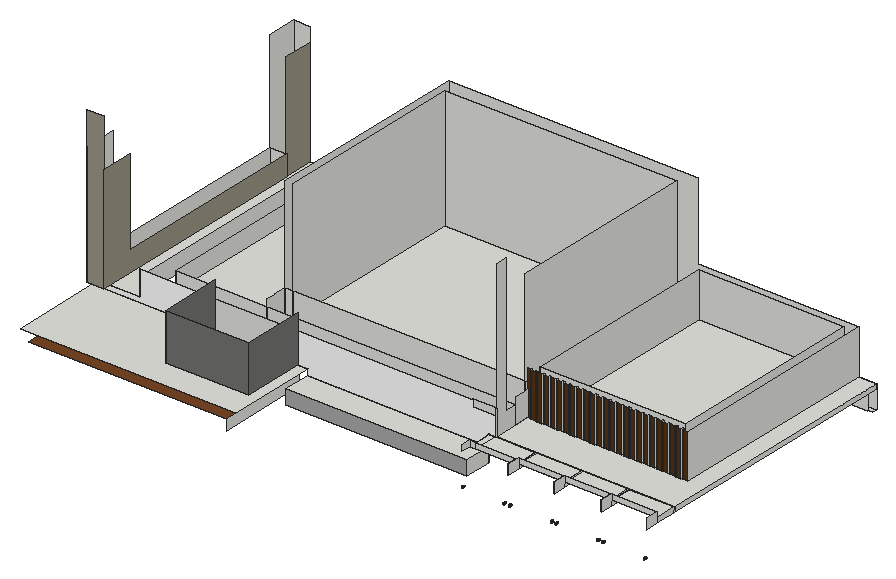
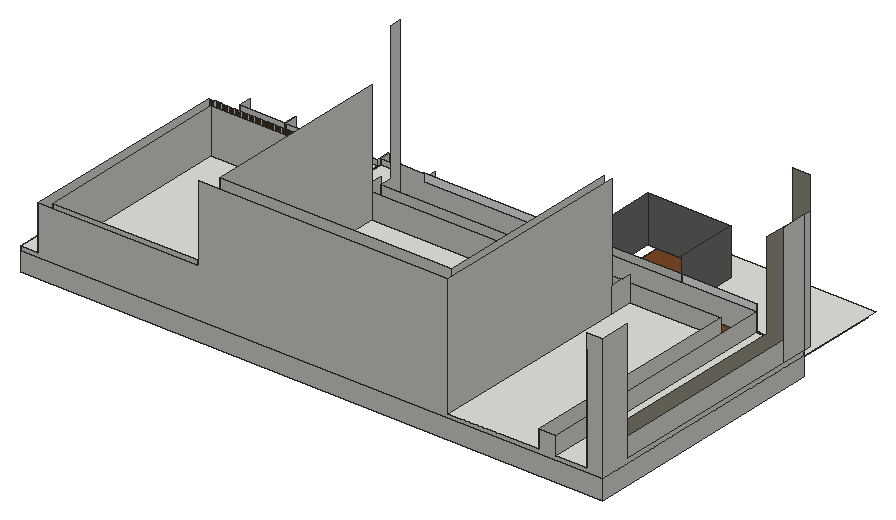
# SketchUp Ruby script. Lengths in inches.
U = 1.inch
M = Sketchup.active_model
def pt(a) = Geom::Point3d.new(a.map { |v| v * U })
def face(e, loops, mat)
  f = e.add_face(loops[0].map { |a| pt(a) })
  loops[1..].each { |l| e.add_face(l.map { |a| pt(a) }).erase! }
  f.material = f.back_material = mat if mat
  f
end
# faces: each face lists its corners as indices into pts; further lists are holes
def faces(e, pts, list, mat = nil) = list.each { |f| face(e, (f[0].is_a?(Array) ? f : [f]).map { |l| l.map { |i| pts[i] } }, mat) }
# xy, xz, yz: faces in a plane at the given z, y or x. An outline is a flat list of corners, or four numbers for a rectangle; further outlines are holes
def ring(l) = l.size == 4 ? [[l[0], l[1]], [l[2], l[1]], [l[2], l[3]], [l[0], l[3]]] : l.each_slice(2).to_a
def flat(e, list, mat, &to3) = list.each { |f| face(e, (f[0].is_a?(Array) ? f : [f]).map { |l| ring(l).map { |u, v| to3.(u, v) } }, mat) }
def xy(e, z, list, mat = nil) = flat(e, list, mat) { |x, y| [x, y, z] }
def xz(e, y, list, mat = nil) = flat(e, list, mat) { |x, z| [x, y, z] }
def yz(e, x, list, mat = nil) = flat(e, list, mat) { |y, z| [x, y, z] }
def lines(e, pts, list) = list.each { |a, b| e.add_line(pt(pts[a]), pt(pts[b])) }
# prism: a flat outline (further loops are holes) pulled along v
def prism(e, loops, v, mat = nil)
  f = face(e, loops, mat); d = Geom::Vector3d.new(v.map { |x| x * U })
  f.pushpull(f.normal.samedirection?(d) ? d.length : -d.length)
end
def box(e, o, s, mat = nil) = prism(e, [[o, [o[0] + s[0], o[1], o[2]], [o[0] + s[0], o[1] + s[1], o[2]], [o[0], o[1] + s[1], o[2]]]], [0, 0, s[2]], mat)
def at(x, y, z, deg = 0) = Geom::Transformation.translation(pt([x, y, z])) * Geom::Transformation.rotation(ORIGIN, Z_AXIS, deg.degrees)
def axes(o, x, y, z) = Geom::Transformation.new([*x, 0, *y, 0, *z, 0, *pt(o).to_a, 1])
def part(name) = M.definitions.add(name)
# library, detail: a bought-in or finely detailed component or shape, given as its bounding box
def library(name, o, s) = part(name).tap { |d| box(d.entities, o, s) }
def detail(e, o, s) = box(e.add_group.entities, o, s)
def put(e, d, t, mat = nil) = e.add_instance(d, t).tap { |i| i.material = mat if mat }
def group(e, t, mat = nil) = e.add_group.tap { |g| g.transformation = t; g.material = mat if mat }.entities
root = M.entities
M.materials.add("[0030_OldLace]").color = [86, 53, 24]
M.materials.add("[0128_White]").color = [255, 255, 255]
M.materials.add("[Color M03]").color = [170, 170, 170]
M.materials.add("[Concrete Tile]").color = [155, 150, 134]
M.materials.add("[Metal Seamed]").color = [116, 117, 113]
M.materials.add("[Wood Veneer 01]").color = [120, 70, 37]
xy(root,95.79,[[684.16,846.1,784.44,851.0625]])
xy(root,99.26,[[621.47,810.97,848.72,845.35]],"[Wood Veneer 01]")
xy(root,101.375,[[545.16,845.35,610.53,846.1],[352.17,846.1,352.17,1160.85,1080.92,1160.85,1080.92,1155.13,357.89,1155.13,357.89,851.0625,545.16,851.0625,545.16,846.1],[545.16,846.1,610.53,851.0625]])
xy(root,101.78,[[374.83,845.35,499.71,851.0625]])
xy(root,114.25,[[363.11,732.28,610.53,845.35]],"[Wood Veneer 01]")
xy(root,117.26,[[621.47,810.97,848.72,845.35]])
xy(root,125.1875,[[352.17,732.28,621.47,732.28,621.47,845.35,609.54,845.35,609.54,767.72,505.35,767.72,505.35,845.35,352.17,845.35],[352.17,845.35,621.47,846.1]])
xy(root,131.1875,[[848.72,814.22,849.1875,844.47],[849.1875,814.22,857.125,844.47],[857.125,814.22,906.77,844.47],[907.71,817.6,964.82,844.47],[965.89,817.6,1022.875,844.47],
  [1024.1875,817.6,1080.92,844.47],[352.17,837.03,372.92,845.35],[848.72,844.47,849.1875,845.35],[849.1875,844.47,857.125,845.35],[857.125,844.47,1080.92,846.1],
  [352.17,845.35,372.92,846.1],[372.92,845.35,411.09,846.1],[848.72,845.35,849.1875,846.1],[849.1875,845.35,857.125,846.1],[352.17,846.1,372.92,877.14],
  [372.92,846.1,411.09,846.1,411.09,1160.85,372.3,1160.85,372.3,1122.97,372.92,1122.97],[857.125,846.1,1080.92,846.1,1080.92,1160.85,1058.5,1160.85,1058.5,893.65,1052.35,893.65,1052.35,895.71,1050.1875,895.71,1050.1875,893.65,1044.04,893.65,1044.04,895.71,1041.875,895.71,1041.875,894.34,1035.73,894.34,1035.73,895.71,1033.5625,895.71,1033.5625,894.34,1027.41,894.34,1027.41,895.71,1025.25,895.71,1025.25,894.34,1019.1,894.34,1019.1,895.71,1016.9375,895.71,1016.9375,894.34,1010.79,894.34,1010.79,895.71,1008.625,895.71,1008.625,894.34,1002.48,894.34,1002.48,895.71,1000.3125,895.71,1000.3125,894.34,994.16,894.34,994.16,895.71,992,895.71,992,894.34,985.85,894.34,985.85,895.71,983.6875,895.71,983.6875,894.34,977.54,894.34,977.54,895.71,975.375,895.71,975.375,894.34,969.23,894.34,969.23,895.71,967.0625,895.71,967.0625,894.34,960.91,894.34,960.91,895.71,958.75,895.71,958.75,894.34,952.6,894.34,952.6,895.71,950.4375,895.71,950.4375,894.34,944.29,894.34,944.29,895.71,942.125,895.71,942.125,894.34,935.98,894.34,935.98,895.71,933.8125,895.71,933.8125,894.34,927.66,894.34,927.66,895.71,925.5,895.71,925.5,894.34,919.35,894.34,919.35,895.71,917.1875,895.71,917.1875,894.34,911.04,894.34,911.04,895.71,908.875,895.71,908.875,894.34,902.73,894.34,902.73,895.71,900.5625,895.71,900.5625,894.34,894.41,894.34,894.41,895.71,892.25,895.71,892.25,894.34,886.1,894.34,886.1,895.71,883.9375,895.71,883.9375,894.34,877.79,894.34,877.79,895.71,875.625,895.71,875.625,894.34,869.48,894.34,869.48,895.71,867.3125,895.71,867.3125,894.34,861.16,894.34,861.16,895.71,857.125,895.71],[352.17,877.14,372.92,1122.97],[431.5,877.14,545.16,1160.85],[545.16,877.14,857.125,905.7],
  [865.59,904.18,1047.28,1152.375],[554.54,905.7,844.86,1143.26]])
xz(root,767.72,[[505.35,125.1875,609.54,183.3125]],"[Metal Seamed]")
xz(root,799.91,[[851.55,91.63,851.84,91.67,852.11,91.78,852.34,91.96,852.52,92.19,852.63,92.46,852.67,92.75,852.63,93.04,852.52,93.32,852.34,93.55,852.11,93.73,851.84,93.84,851.55,93.88,851.25,93.84,850.98,93.73,850.75,93.55,850.57,93.32,850.46,93.04,850.42,92.75,850.46,92.46,850.57,92.19,850.75,91.96,850.98,91.78,851.25,91.67],[903.73,91.63,904.02,91.67,904.3,91.78,904.53,91.96,904.71,92.19,904.82,92.46,904.86,92.75,904.82,93.04,904.71,93.32,904.53,93.55,904.3,93.73,904.02,93.84,903.73,93.88,903.44,93.84,903.17,93.73,902.9375,93.55,902.76,93.32,902.65,93.04,902.61,92.75,902.65,92.46,902.76,92.19,902.9375,91.96,903.17,91.78,903.44,91.67],[910.53,91.63,910.82,91.67,911.1,91.78,911.33,91.96,911.51,92.19,911.62,92.46,911.66,92.75,911.62,93.04,911.51,93.32,911.33,93.55,911.1,93.73,910.82,93.84,910.53,93.88,910.24,93.84,909.97,93.73,909.74,93.55,909.56,93.32,909.45,93.04,909.41,92.75,909.45,92.46,909.56,92.19,909.74,91.96,909.97,91.78,910.24,91.67],[962.72,91.63,963.01,91.67,963.28,91.78,963.52,91.96,963.7,92.19,963.81,92.46,963.85,92.75,963.81,93.04,963.7,93.32,963.52,93.55,963.28,93.73,963.01,93.84,962.72,93.88,962.43,93.84,962.16,93.73,961.93,93.55,961.75,93.32,961.63,93.04,961.6,92.75,961.63,92.46,961.75,92.19,961.93,91.96,962.16,91.78,962.43,91.67],[968.71,91.63,969,91.67,969.27,91.78,969.5,91.96,969.68,92.19,969.8,92.46,969.83,92.75,969.8,93.04,969.68,93.32,969.5,93.55,969.27,93.73,969,93.84,968.71,93.88,968.42,93.84,968.15,93.73,967.91,93.55,967.74,93.32,967.62,93.04,967.58,92.75,967.62,92.46,967.74,92.19,967.91,91.96,968.15,91.78,968.42,91.67],
  [1020.9,91.63,1021.1875,91.67,1021.46,91.78,1021.69,91.96,1021.87,92.19,1021.98,92.46,1022.02,92.75,1021.98,93.04,1021.87,93.32,1021.69,93.55,1021.46,93.73,1021.1875,93.84,1020.9,93.88,1020.61,93.84,1020.33,93.73,1020.1,93.55,1019.92,93.32,1019.81,93.04,1019.77,92.75,1019.81,92.46,1019.92,92.19,1020.1,91.96,1020.33,91.78,1020.61,91.67],[1027.01,91.63,1027.3,91.67,1027.57,91.78,1027.81,91.96,1027.98,92.19,1028.1,92.46,1028.14,92.75,1028.1,93.04,1027.98,93.32,1027.81,93.55,1027.57,93.73,1027.3,93.84,1027.01,93.88,1026.72,93.84,1026.45,93.73,1026.21,93.55,1026.04,93.32,1025.92,93.04,1025.89,92.75,1025.92,92.46,1026.04,92.19,1026.21,91.96,1026.45,91.78,1026.72,91.67],[1079.2,91.63,1079.49,91.67,1079.76,91.78,1079.99,91.96,1080.17,92.19,1080.28,92.46,1080.32,92.75,1080.28,93.04,1080.17,93.32,1079.99,93.55,1079.76,93.73,1079.49,93.84,1079.2,93.88,1078.91,93.84,1078.64,93.73,1078.4,93.55,1078.22,93.32,1078.11,93.04,1078.07,92.75,1078.11,92.46,1078.22,92.19,1078.4,91.96,1078.64,91.78,1078.91,91.67]])
xz(root,810.97,[[621.47,99.26,848.72,117.26]],"[Color M03]")
xz(root,814.22,[[848.72,131.1875,857.125,138.0625],[857.125,131.1875,906.77,138.0625]])
xz(root,817.6,[[907.71,131.1875,964.82,138.0625],[965.89,131.1875,1022.875,138.0625],[1024.1875,131.1875,1080.92,138.0625]])
xz(root,837.03,[[352.17,131.1875,372.92,324.5625]],"[Concrete Tile]")
xz(root,845.35,[[621.47,99.26,848.72,117.26],[505.35,125.1875,609.54,162.75]])
xz(root,845.35,[[621.47,117.26,848.72,117.26,848.72,131.1875,857.125,131.1875,857.125,154.75,827.91,154.75,827.91,162.75,609.54,162.75,609.54,125.1875,621.47,125.1875],[352.17,125.1875,505.35,125.1875,505.35,162.75,411.09,162.75,411.09,131.1875,352.17,131.1875]],"[0128_White]")
xz(root,846.1,[[352.17,125.1875,352.17,131.1875,411.09,131.1875,411.09,153.5625,827.91,153.5625,827.91,163,857.125,163,857.125,131.1875,848.72,131.1875,848.72,125.1875]])
xz(root,851.0625,[[374.83,101.375,499.71,101.78]])
xz(root,877.14,[[431.5,131.1875,545.16,153.5625],[545.16,131.1875,857.125,153.5625]])
xz(root,893.65,[[1044.04,131.1875,1050.1875,186.75],[1052.35,131.1875,1058.5,186.75]],"[0030_OldLace]")
xz(root,894.34,[[861.16,131.1875,867.3125,186.75],[869.48,131.1875,875.625,186.75],[877.79,131.1875,883.9375,186.75],[886.1,131.1875,892.25,186.75],[894.41,131.1875,900.5625,186.75],
  [902.73,131.1875,908.875,186.75],[911.04,131.1875,917.1875,186.75],[919.35,131.1875,925.5,186.75],[927.66,131.1875,933.8125,186.75],[935.98,131.1875,942.125,186.75],
  [944.29,131.1875,950.4375,186.75],[952.6,131.1875,958.75,186.75],[960.91,131.1875,967.0625,186.75],[969.23,131.1875,975.375,186.75],[977.54,131.1875,983.6875,186.75],
  [985.85,131.1875,992,186.75],[994.16,131.1875,1000.3125,186.75],[1002.48,131.1875,1008.625,186.75],[1010.79,131.1875,1016.9375,186.75],[1019.1,131.1875,1025.25,186.75],
  [1027.41,131.1875,1033.5625,186.75],[1035.73,131.1875,1041.875,186.75]],"[0030_OldLace]")
xz(root,895.71,[[857.125,131.1875,861.16,186.75],[867.3125,131.1875,869.48,186.75],[875.625,131.1875,877.79,186.75],[883.9375,131.1875,886.1,186.75],[892.25,131.1875,894.41,186.75],
  [900.5625,131.1875,902.73,186.75],[908.875,131.1875,911.04,186.75],[917.1875,131.1875,919.35,186.75],[925.5,131.1875,927.66,186.75],[933.8125,131.1875,935.98,186.75],
  [942.125,131.1875,944.29,186.75],[950.4375,131.1875,952.6,186.75],[958.75,131.1875,960.91,186.75],[967.0625,131.1875,969.23,186.75],[975.375,131.1875,977.54,186.75],
  [983.6875,131.1875,985.85,186.75],[992,131.1875,994.16,186.75],[1000.3125,131.1875,1002.48,186.75],[1008.625,131.1875,1010.79,186.75],[1016.9375,131.1875,1019.1,186.75],
  [1025.25,131.1875,1027.41,186.75],[1033.5625,131.1875,1035.73,186.75],[1041.875,131.1875,1044.04,186.75],[1050.1875,131.1875,1052.35,186.75]],"[0030_OldLace]")
xz(root,904.18,[[865.59,131.1875,1047.28,186.75]])
xz(root,905.7,[[545.16,131.1875,554.54,162.75],[554.54,131.1875,844.86,162.75],[844.86,131.1875,857.125,162.75]])
xz(root,1122.97,[[352.17,131.1875,372.3,156.5],[372.3,131.1875,372.92,156.5]])
xz(root,1143.26,[[554.54,131.1875,844.86,282.75]])
xz(root,1152.375,[[865.59,131.1875,1047.28,186.75]])
xz(root,1155.13,[[357.89,101.375,1075.21,125.1875]])
xz(root,1160.85,[[352.17,101.375,1080.92,125.1875],[352.17,125.1875,352.17,282.75,372.3,282.75,372.3,131.1875,411.09,131.1875,411.09,153.5625,431.5,153.5625,431.5,131.1875,545.16,131.1875,545.16,282.75,857.125,282.75,857.125,186.75,1058.5,186.75,1058.5,131.1875,1080.92,131.1875,1080.92,125.1875]])
yz(root,352.17,[[846.1,101.375,1160.85,125.1875],[845.35,125.1875,846.1,131.1875],[846.1,125.1875,846.1,131.1875,1122.97,131.1875,1122.97,282.75,1160.85,282.75,1160.85,125.1875],[837.03,131.1875,845.35,282.75],[845.35,131.1875,877.14,282.75],
  [877.14,131.1875,1122.97,156.5]])
yz(root,357.89,[[851.0625,101.375,1155.13,125.1875]])
yz(root,372.3,[[1122.97,131.1875,1160.85,264.75]],"[Concrete Tile]")
yz(root,372.92,[[837.03,131.1875,1122.97,131.1875,1122.97,156.5,877.14,156.5,877.14,264.75,837.03,264.75]],"[Concrete Tile]")
yz(root,411.09,[[845.35,131.1875,846.1,162.75],[846.1,131.1875,1160.85,153.5625]])
yz(root,431.5,[[877.14,131.1875,1160.85,153.5625]])
yz(root,505.35,[[767.72,125.1875,845.35,183.3125]],"[Metal Seamed]")
yz(root,545.16,[[877.14,131.1875,877.14,162.125,888.95,162.125,888.95,162.75,905.7,162.75,905.7,131.1875],[905.7,131.1875,1160.85,282.75]])
yz(root,554.54,[[905.7,131.1875,1143.26,282.75]])
yz(root,609.54,[[767.72,125.1875,845.35,183.3125]],"[Metal Seamed]")
yz(root,610.53,[[732.28,101.375,845.35,114.25]])
yz(root,844.86,[[905.7,131.1875,1143.26,282.75]])
yz(root,848.72,[[810.97,99.26,844.47,117.26],[844.47,99.26,845.35,117.26],[844.47,117.26,845.35,125.1875],[844.47,125.1875,845.35,131.1875],[845.35,125.1875,846.1,131.1875],
  [801.78,131.1875,814.22,138.0625]])
yz(root,857.125,[[845.35,131.1875,846.1,163],[846.1,131.1875,877.14,131.1875,877.14,153.5625,861.24,153.5625,861.24,324.5625,846.1,324.5625],[877.14,131.1875,895.71,131.1875,895.71,162.75,890.39,162.75,890.39,162.125,877.14,162.125],[895.71,131.1875,905.7,162.75]])
yz(root,861.16,[[894.34,131.1875,895.71,186.75]])
yz(root,865.59,[[904.18,131.1875,905.7,186.75],[905.7,131.1875,1152.375,186.75]])
yz(root,867.3125,[[894.34,131.1875,895.71,186.75]])
yz(root,869.48,[[894.34,131.1875,895.71,186.75]])
yz(root,875.625,[[894.34,131.1875,895.71,186.75]])
yz(root,877.79,[[894.34,131.1875,895.71,186.75]])
yz(root,883.9375,[[894.34,131.1875,895.71,186.75]])
yz(root,886.1,[[894.34,131.1875,895.71,186.75]])
yz(root,892.25,[[894.34,131.1875,895.71,186.75]])
yz(root,894.41,[[894.34,131.1875,895.71,186.75]])
yz(root,900.5625,[[894.34,131.1875,895.71,186.75]])
yz(root,902.73,[[894.34,131.1875,895.71,186.75]])
yz(root,906.77,[[801.78,125.1875,814.22,138.0625],[814.22,125.1875,844.47,131.1875]])
yz(root,907.71,[[801.78,125.1875,817.6,138.0625],[817.6,125.1875,844.47,131.1875]])
yz(root,908.875,[[894.34,131.1875,895.71,186.75]])
yz(root,911.04,[[894.34,131.1875,895.71,186.75]])
yz(root,917.1875,[[894.34,131.1875,895.71,186.75]])
yz(root,919.35,[[894.34,131.1875,895.71,186.75]])
yz(root,925.5,[[894.34,131.1875,895.71,186.75]])
yz(root,927.66,[[894.34,131.1875,895.71,186.75]])
yz(root,933.8125,[[894.34,131.1875,895.71,186.75]])
yz(root,935.98,[[894.34,131.1875,895.71,186.75]])
yz(root,942.125,[[894.34,131.1875,895.71,186.75]])
yz(root,944.29,[[894.34,131.1875,895.71,186.75]])
yz(root,950.4375,[[894.34,131.1875,895.71,186.75]])
yz(root,952.6,[[894.34,131.1875,895.71,186.75]])
yz(root,958.75,[[894.34,131.1875,895.71,186.75]])
yz(root,960.91,[[894.34,131.1875,895.71,186.75]])
yz(root,964.82,[[801.78,125.1875,817.6,138.0625],[817.6,125.1875,844.47,131.1875]])
yz(root,965.89,[[801.78,125.1875,817.6,138.0625],[817.6,125.1875,844.47,131.1875]])
yz(root,967.0625,[[894.34,131.1875,895.71,186.75]])
yz(root,969.23,[[894.34,131.1875,895.71,186.75]])
yz(root,975.375,[[894.34,131.1875,895.71,186.75]])
yz(root,977.54,[[894.34,131.1875,895.71,186.75]])
yz(root,983.6875,[[894.34,131.1875,895.71,186.75]])
yz(root,985.85,[[894.34,131.1875,895.71,186.75]])
yz(root,992,[[894.34,131.1875,895.71,186.75]])
yz(root,994.16,[[894.34,131.1875,895.71,186.75]])
yz(root,1000.3125,[[894.34,131.1875,895.71,186.75]])
yz(root,1002.48,[[894.34,131.1875,895.71,186.75]])
yz(root,1008.625,[[894.34,131.1875,895.71,186.75]])
yz(root,1010.79,[[894.34,131.1875,895.71,186.75]])
yz(root,1016.9375,[[894.34,131.1875,895.71,186.75]])
yz(root,1019.1,[[894.34,131.1875,895.71,186.75]])
yz(root,1022.875,[[801.78,125.1875,817.6,138.0625],[817.6,125.1875,844.47,131.1875]])
yz(root,1024.1875,[[801.78,125.1875,817.6,138.0625],[817.6,125.1875,844.47,131.1875]])
yz(root,1025.25,[[894.34,131.1875,895.71,186.75]])
yz(root,1027.41,[[894.34,131.1875,895.71,186.75]])
yz(root,1033.5625,[[894.34,131.1875,895.71,186.75]])
yz(root,1035.73,[[894.34,131.1875,895.71,186.75]],"[0030_OldLace]")
yz(root,1041.875,[[894.34,131.1875,895.71,186.75]])
yz(root,1044.04,[[893.65,131.1875,895.71,186.75]],"[0030_OldLace]")
yz(root,1047.28,[[904.18,131.1875,1152.375,186.75]])
yz(root,1050.1875,[[893.65,131.1875,895.71,186.75]])
yz(root,1052.35,[[893.65,131.1875,895.71,186.75]],"[0030_OldLace]")
yz(root,1058.5,[[893.65,131.1875,1160.85,186.75]])
yz(root,1080.92,[[801.78,125.1875,817.6,138.0625],[817.6,125.1875,844.47,131.1875],[844.47,125.1875,846.1,131.1875],[846.1,125.1875,1160.85,131.1875]])
p = [[851.25,801.78,91.67],[851.55,801.78,91.63],[851.55,799.91,91.63],[851.25,799.91,91.67],[851.84,801.78,91.67],[851.84,799.91,91.67],
  [903.44,801.78,91.67],[903.73,801.78,91.63],[903.73,799.91,91.63],[903.44,799.91,91.67],[904.02,801.78,91.67],[904.02,799.91,91.67],
  [910.24,801.78,91.67],[910.53,801.78,91.63],[910.53,799.91,91.63],[910.24,799.91,91.67],[910.82,801.78,91.67],[910.82,799.91,91.67],
  [962.43,801.78,91.67],[962.72,801.78,91.63],[962.72,799.91,91.63],[962.43,799.91,91.67],[963.01,801.78,91.67],[963.01,799.91,91.67],
  [968.42,801.78,91.67],[968.71,801.78,91.63],[968.71,799.91,91.63],[968.42,799.91,91.67],[969,801.78,91.67],[969,799.91,91.67],
  [1020.61,801.78,91.67],[1020.9,801.78,91.63],[1020.9,799.91,91.63],[1020.61,799.91,91.67],[1021.1875,801.78,91.67],[1021.1875,799.91,91.67],
  [1026.72,801.78,91.67],[1027.01,801.78,91.63],[1027.01,799.91,91.63],[1026.72,799.91,91.67],[1027.3,801.78,91.67],[1027.3,799.91,91.67],
  [1078.91,801.78,91.67],[1079.2,801.78,91.63],[1079.2,799.91,91.63],[1078.91,799.91,91.67],[1079.49,801.78,91.67],[1079.49,799.91,91.67],
  [850.98,801.78,91.78],[850.98,799.91,91.78],[852.11,801.78,91.78],[852.11,799.91,91.78],[903.17,801.78,91.78],[903.17,799.91,91.78],
  [904.3,801.78,91.78],[904.3,799.91,91.78],[909.97,801.78,91.78],[909.97,799.91,91.78],[911.1,801.78,91.78],[911.1,799.91,91.78],
  [962.16,801.78,91.78],[962.16,799.91,91.78],[963.28,801.78,91.78],[963.28,799.91,91.78],[968.15,801.78,91.78],[968.15,799.91,91.78],
  [969.27,801.78,91.78],[969.27,799.91,91.78],[1020.33,801.78,91.78],[1020.33,799.91,91.78],[1021.46,801.78,91.78],[1021.46,799.91,91.78],
  [1026.45,801.78,91.78],[1026.45,799.91,91.78],[1027.57,801.78,91.78],[1027.57,799.91,91.78],[1078.64,801.78,91.78],[1078.64,799.91,91.78],
  [1079.76,801.78,91.78],[1079.76,799.91,91.78],[850.75,801.78,91.96],[850.75,799.91,91.96],[852.34,801.78,91.96],[852.34,799.91,91.96],
  [902.9375,801.78,91.96],[902.9375,799.91,91.96],[904.53,801.78,91.96],[904.53,799.91,91.96],[909.74,801.78,91.96],[909.74,799.91,91.96],
  [911.33,801.78,91.96],[911.33,799.91,91.96],[961.93,801.78,91.96],[961.93,799.91,91.96],[963.52,801.78,91.96],[963.52,799.91,91.96],
  [967.91,801.78,91.96],[967.91,799.91,91.96],[969.5,801.78,91.96],[969.5,799.91,91.96],[1020.1,801.78,91.96],[1020.1,799.91,91.96],
  [1021.69,801.78,91.96],[1021.69,799.91,91.96],[1026.21,801.78,91.96],[1026.21,799.91,91.96],[1027.81,801.78,91.96],[1027.81,799.91,91.96],
  [1078.4,801.78,91.96],[1078.4,799.91,91.96],[1079.99,801.78,91.96],[1079.99,799.91,91.96],[850.57,801.78,92.19],[850.57,799.91,92.19],
  [852.52,801.78,92.19],[852.52,799.91,92.19],[902.76,801.78,92.19],[902.76,799.91,92.19],[904.71,801.78,92.19],[904.71,799.91,92.19],
  [909.56,801.78,92.19],[909.56,799.91,92.19],[911.51,801.78,92.19],[911.51,799.91,92.19],[961.75,801.78,92.19],[961.75,799.91,92.19],
  [963.7,801.78,92.19],[963.7,799.91,92.19],[967.74,801.78,92.19],[967.74,799.91,92.19],[969.68,801.78,92.19],[969.68,799.91,92.19],
  [1019.92,801.78,92.19],[1019.92,799.91,92.19],[1021.87,801.78,92.19],[1021.87,799.91,92.19],[1026.04,801.78,92.19],[1026.04,799.91,92.19],
  [1027.98,801.78,92.19],[1027.98,799.91,92.19],[1078.22,801.78,92.19],[1078.22,799.91,92.19],[1080.17,801.78,92.19],[1080.17,799.91,92.19],
  [850.46,801.78,92.46],[850.46,799.91,92.46],[852.63,801.78,92.46],[852.63,799.91,92.46],[902.65,801.78,92.46],[902.65,799.91,92.46],
  [904.82,801.78,92.46],[904.82,799.91,92.46],[909.45,801.78,92.46],[909.45,799.91,92.46],[911.62,801.78,92.46],[911.62,799.91,92.46],
  [961.63,801.78,92.46],[961.63,799.91,92.46],[963.81,801.78,92.46],[963.81,799.91,92.46],[967.62,801.78,92.46],[967.62,799.91,92.46],
  [969.8,801.78,92.46],[969.8,799.91,92.46],[1019.81,801.78,92.46],[1019.81,799.91,92.46],[1021.98,801.78,92.46],[1021.98,799.91,92.46],
  [1025.92,801.78,92.46],[1025.92,799.91,92.46],[1028.1,801.78,92.46],[1028.1,799.91,92.46],[1078.11,801.78,92.46],[1078.11,799.91,92.46],
  [1080.28,801.78,92.46],[1080.28,799.91,92.46],[850.42,801.78,92.75],[850.42,799.91,92.75],[852.67,801.78,92.75],[852.67,799.91,92.75],
  [902.61,801.78,92.75],[902.61,799.91,92.75],[904.86,801.78,92.75],[904.86,799.91,92.75],[909.41,801.78,92.75],[909.41,799.91,92.75],
  [911.66,801.78,92.75],[911.66,799.91,92.75],[961.6,801.78,92.75],[961.6,799.91,92.75],[963.85,801.78,92.75],[963.85,799.91,92.75],
  [967.58,801.78,92.75],[967.58,799.91,92.75],[969.83,801.78,92.75],[969.83,799.91,92.75],[1019.77,801.78,92.75],[1019.77,799.91,92.75],
  [1022.02,801.78,92.75],[1022.02,799.91,92.75],[1025.89,801.78,92.75],[1025.89,799.91,92.75],[1028.14,801.78,92.75],[1028.14,799.91,92.75],
  [1078.07,801.78,92.75],[1078.07,799.91,92.75],[1080.32,801.78,92.75],[1080.32,799.91,92.75],[850.46,801.78,93.04],[850.46,799.91,93.04],
  [852.63,801.78,93.04],[852.63,799.91,93.04],[902.65,801.78,93.04],[902.65,799.91,93.04],[904.82,801.78,93.04],[904.82,799.91,93.04],
  [909.45,801.78,93.04],[909.45,799.91,93.04],[911.62,801.78,93.04],[911.62,799.91,93.04],[961.63,801.78,93.04],[961.63,799.91,93.04],
  [963.81,801.78,93.04],[963.81,799.91,93.04],[967.62,801.78,93.04],[967.62,799.91,93.04],[969.8,801.78,93.04],[969.8,799.91,93.04],
  [1019.81,801.78,93.04],[1019.81,799.91,93.04],[1021.98,801.78,93.04],[1021.98,799.91,93.04],[1025.92,801.78,93.04],[1025.92,799.91,93.04],
  [1028.1,801.78,93.04],[1028.1,799.91,93.04],[1078.11,801.78,93.04],[1078.11,799.91,93.04],[1080.28,801.78,93.04],[1080.28,799.91,93.04],
  [850.57,801.78,93.32],[850.57,799.91,93.32],[852.52,801.78,93.32],[852.52,799.91,93.32],[902.76,801.78,93.32],[902.76,799.91,93.32],
  [904.71,801.78,93.32],[904.71,799.91,93.32],[909.56,801.78,93.32],[909.56,799.91,93.32],[911.51,801.78,93.32],[911.51,799.91,93.32],
  [961.75,801.78,93.32],[961.75,799.91,93.32],[963.7,801.78,93.32],[963.7,799.91,93.32],[967.74,801.78,93.32],[967.74,799.91,93.32],
  [969.68,801.78,93.32],[969.68,799.91,93.32],[1019.92,801.78,93.32],[1019.92,799.91,93.32],[1021.87,801.78,93.32],[1021.87,799.91,93.32],
  [1026.04,801.78,93.32],[1026.04,799.91,93.32],[1027.98,801.78,93.32],[1027.98,799.91,93.32],[1078.22,801.78,93.32],[1078.22,799.91,93.32],
  [1080.17,801.78,93.32],[1080.17,799.91,93.32],[850.75,801.78,93.55],[850.75,799.91,93.55],[852.34,801.78,93.55],[852.34,799.91,93.55],
  [902.9375,801.78,93.55],[902.9375,799.91,93.55],[904.53,801.78,93.55],[904.53,799.91,93.55],[909.74,801.78,93.55],[909.74,799.91,93.55],
  [911.33,801.78,93.55],[911.33,799.91,93.55],[961.93,801.78,93.55],[961.93,799.91,93.55],[963.52,801.78,93.55],[963.52,799.91,93.55],
  [967.91,801.78,93.55],[967.91,799.91,93.55],[969.5,801.78,93.55],[969.5,799.91,93.55],[1020.1,801.78,93.55],[1020.1,799.91,93.55],
  [1021.69,801.78,93.55],[1021.69,799.91,93.55],[1026.21,801.78,93.55],[1026.21,799.91,93.55],[1027.81,801.78,93.55],[1027.81,799.91,93.55],
  [1078.4,801.78,93.55],[1078.4,799.91,93.55],[1079.99,801.78,93.55],[1079.99,799.91,93.55],[850.98,801.78,93.73],[850.98,799.91,93.73],
  [852.11,801.78,93.73],[852.11,799.91,93.73],[903.17,801.78,93.73],[903.17,799.91,93.73],[904.3,801.78,93.73],[904.3,799.91,93.73],
  [909.97,801.78,93.73],[909.97,799.91,93.73],[911.1,801.78,93.73],[911.1,799.91,93.73],[962.16,801.78,93.73],[962.16,799.91,93.73],
  [963.28,801.78,93.73],[963.28,799.91,93.73],[968.15,801.78,93.73],[968.15,799.91,93.73],[969.27,801.78,93.73],[969.27,799.91,93.73],
  [1020.33,801.78,93.73],[1020.33,799.91,93.73],[1021.46,801.78,93.73],[1021.46,799.91,93.73],[1026.45,801.78,93.73],[1026.45,799.91,93.73],
  [1027.57,801.78,93.73],[1027.57,799.91,93.73],[1078.64,801.78,93.73],[1078.64,799.91,93.73],[1079.76,801.78,93.73],[1079.76,799.91,93.73],
  [851.25,801.78,93.84],[851.25,799.91,93.84],[851.84,801.78,93.84],[851.84,799.91,93.84],[903.44,801.78,93.84],[903.44,799.91,93.84],
  [904.02,801.78,93.84],[904.02,799.91,93.84],[910.24,801.78,93.84],[910.24,799.91,93.84],[910.82,801.78,93.84],[910.82,799.91,93.84],
  [962.43,801.78,93.84],[962.43,799.91,93.84],[963.01,801.78,93.84],[963.01,799.91,93.84],[968.42,801.78,93.84],[968.42,799.91,93.84],
  [969,801.78,93.84],[969,799.91,93.84],[1020.61,801.78,93.84],[1020.61,799.91,93.84],[1021.1875,801.78,93.84],[1021.1875,799.91,93.84],
  [1026.72,801.78,93.84],[1026.72,799.91,93.84],[1027.3,801.78,93.84],[1027.3,799.91,93.84],[1078.91,801.78,93.84],[1078.91,799.91,93.84],
  [1079.49,801.78,93.84],[1079.49,799.91,93.84],[851.55,801.78,93.88],[851.55,799.91,93.88],[903.73,801.78,93.88],[903.73,799.91,93.88],
  [910.53,801.78,93.88],[910.53,799.91,93.88],[962.72,801.78,93.88],[962.72,799.91,93.88],[968.71,801.78,93.88],[968.71,799.91,93.88],
  [1020.9,801.78,93.88],[1020.9,799.91,93.88],[1027.01,801.78,93.88],[1027.01,799.91,93.88],[1079.2,801.78,93.88],[1079.2,799.91,93.88]]
faces(root,p,[[0,1,2,3],[1,4,5,2],[6,7,8,9],[7,10,11,8],[12,13,14,15],[13,16,17,14],[18,19,20,21],[19,22,23,20],
  [24,25,26,27],[25,28,29,26],[30,31,32,33],[31,34,35,32],[36,37,38,39],[37,40,41,38],[42,43,44,45],[43,46,47,44],
  [48,0,3,49],[4,50,51,5],[52,6,9,53],[10,54,55,11],[56,12,15,57],[16,58,59,17],[60,18,21,61],[22,62,63,23],
  [64,24,27,65],[28,66,67,29],[68,30,33,69],[34,70,71,35],[72,36,39,73],[40,74,75,41],[76,42,45,77],[46,78,79,47],
  [80,48,49,81],[50,82,83,51],[84,52,53,85],[54,86,87,55],[88,56,57,89],[58,90,91,59],[92,60,61,93],[62,94,95,63],
  [96,64,65,97],[66,98,99,67],[100,68,69,101],[70,102,103,71],[104,72,73,105],[74,106,107,75],[108,76,77,109],[78,110,111,79],
  [112,80,81,113],[82,114,115,83],[116,84,85,117],[86,118,119,87],[120,88,89,121],[90,122,123,91],[124,92,93,125],[94,126,127,95],
  [128,96,97,129],[98,130,131,99],[132,100,101,133],[102,134,135,103],[136,104,105,137],[106,138,139,107],[140,108,109,141],[110,142,143,111],
  [144,112,113,145],[114,146,147,115],[148,116,117,149],[118,150,151,119],[152,120,121,153],[122,154,155,123],[156,124,125,157],[126,158,159,127],
  [160,128,129,161],[130,162,163,131],[164,132,133,165],[134,166,167,135],[168,136,137,169],[138,170,171,139],[172,140,141,173],[142,174,175,143],
  [176,144,145,177],[146,178,179,147],[180,148,149,181],[150,182,183,151],[184,152,153,185],[154,186,187,155],[188,156,157,189],[158,190,191,159],
  [192,160,161,193],[162,194,195,163],[196,164,165,197],[166,198,199,167],[200,168,169,201],[170,202,203,171],[204,172,173,205],[174,206,207,175],
  [208,176,177,209],[178,210,211,179],[212,180,181,213],[182,214,215,183],[216,184,185,217],[186,218,219,187],[220,188,189,221],[190,222,223,191],
  [224,192,193,225],[194,226,227,195],[228,196,197,229],[198,230,231,199],[232,200,201,233],[202,234,235,203],[236,204,205,237],[206,238,239,207],
  [240,208,209,241],[210,242,243,211],[244,212,213,245],[214,246,247,215],[248,216,217,249],[218,250,251,219],[252,220,221,253],[222,254,255,223],
  [256,224,225,257],[226,258,259,227],[260,228,229,261],[230,262,263,231],[264,232,233,265],[234,266,267,235],[268,236,237,269],[238,270,271,239],
  [272,240,241,273],[242,274,275,243],[276,244,245,277],[246,278,279,247],[280,248,249,281],[250,282,283,251],[284,252,253,285],[254,286,287,255],
  [288,256,257,289],[258,290,291,259],[292,260,261,293],[262,294,295,263],[296,264,265,297],[266,298,299,267],[300,268,269,301],[270,302,303,271],
  [304,272,273,305],[274,306,307,275],[308,276,277,309],[278,310,311,279],[312,280,281,313],[282,314,315,283],[316,284,285,317],[286,318,319,287],
  [320,288,289,321],[290,322,323,291],[324,292,293,325],[294,326,327,295],[328,296,297,329],[298,330,331,299],[332,300,301,333],[302,334,335,303],
  [336,304,305,337],[306,338,339,307],[340,308,309,341],[310,342,343,311],[344,312,313,345],[314,346,347,315],[348,316,317,349],[318,350,351,319],
  [352,320,321,353],[322,354,355,323],[356,324,325,357],[326,358,359,327],[360,328,329,361],[330,362,363,331],[364,332,333,365],[334,366,367,335],
  [368,336,337,369],[338,368,369,339],[370,340,341,371],[342,370,371,343],[372,344,345,373],[346,372,373,347],[374,348,349,375],[350,374,375,351],
  [376,352,353,377],[354,376,377,355],[378,356,357,379],[358,378,379,359],[380,360,361,381],[362,380,381,363],[382,364,365,383],[366,382,383,367]])
